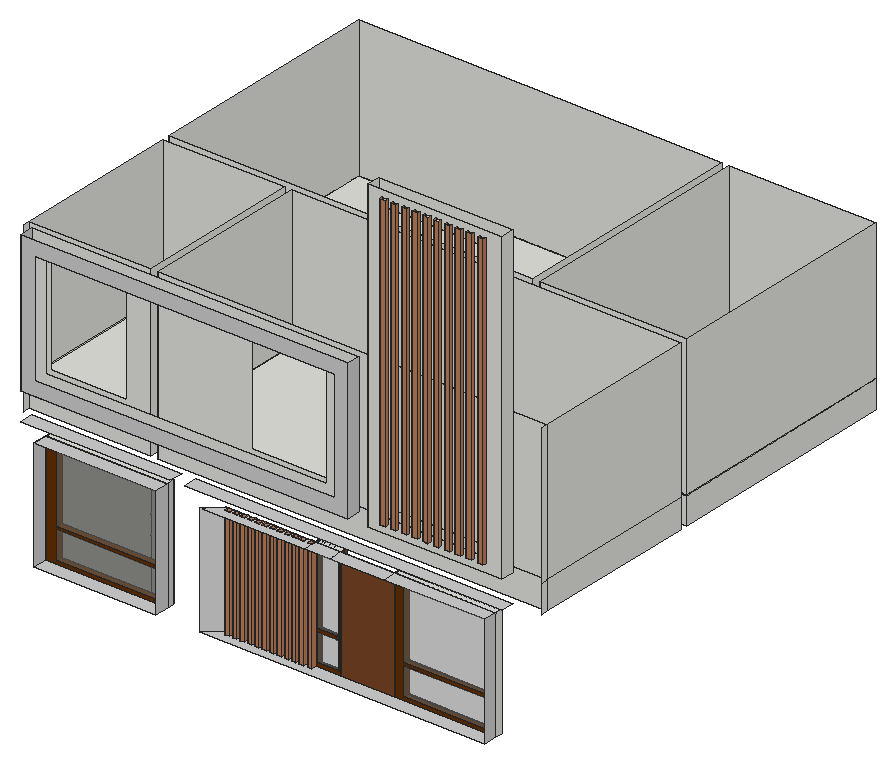
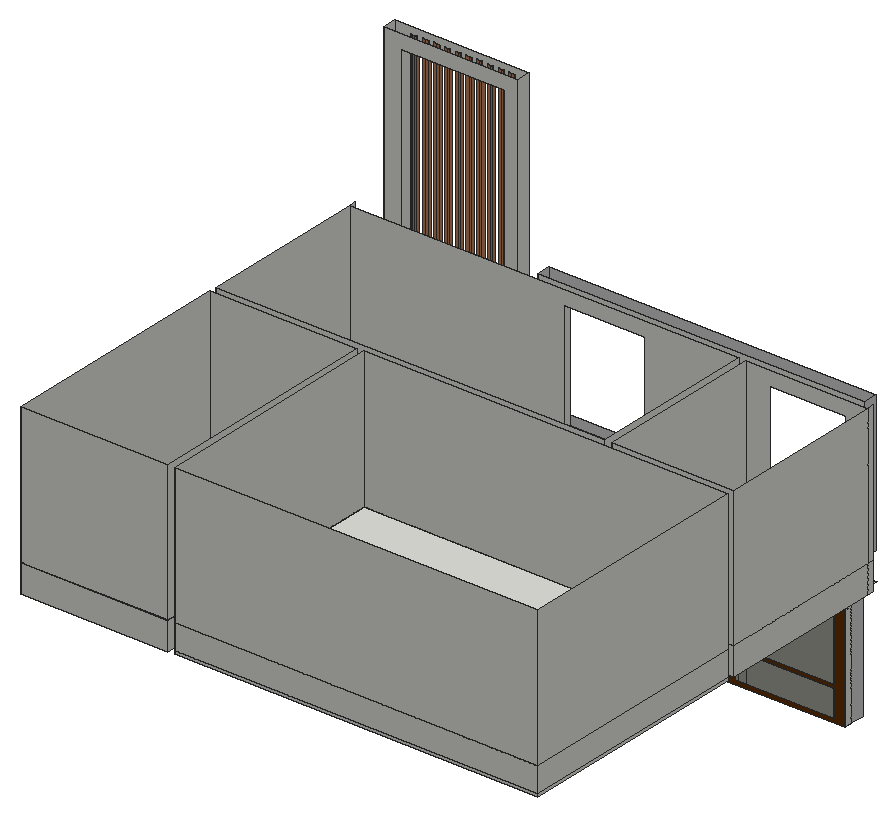
# SketchUp Ruby script. Lengths in inches.
U = 1.inch
M = Sketchup.active_model
def pt(a) = Geom::Point3d.new(a.map { |v| v * U })
def face(e, loops, mat)
  f = e.add_face(loops[0].map { |a| pt(a) })
  loops[1..].each { |l| e.add_face(l.map { |a| pt(a) }).erase! }
  f.material = f.back_material = mat if mat
  f
end
# faces: each face lists its corners as indices into pts; further lists are holes
def faces(e, pts, list, mat = nil) = list.each { |f| face(e, (f[0].is_a?(Array) ? f : [f]).map { |l| l.map { |i| pts[i] } }, mat) }
# xy, xz, yz: faces in a plane at the given z, y or x. An outline is a flat list of corners, or four numbers for a rectangle; further outlines are holes
def ring(l) = l.size == 4 ? [[l[0], l[1]], [l[2], l[1]], [l[2], l[3]], [l[0], l[3]]] : l.each_slice(2).to_a
def flat(e, list, mat, &to3) = list.each { |f| face(e, (f[0].is_a?(Array) ? f : [f]).map { |l| ring(l).map { |u, v| to3.(u, v) } }, mat) }
def xy(e, z, list, mat = nil) = flat(e, list, mat) { |x, y| [x, y, z] }
def xz(e, y, list, mat = nil) = flat(e, list, mat) { |x, z| [x, y, z] }
def yz(e, x, list, mat = nil) = flat(e, list, mat) { |y, z| [x, y, z] }
def lines(e, pts, list) = list.each { |a, b| e.add_line(pt(pts[a]), pt(pts[b])) }
# prism: a flat outline (further loops are holes) pulled along v
def prism(e, loops, v, mat = nil)
  f = face(e, loops, mat); d = Geom::Vector3d.new(v.map { |x| x * U })
  f.pushpull(f.normal.samedirection?(d) ? d.length : -d.length)
end
def box(e, o, s, mat = nil) = prism(e, [[o, [o[0] + s[0], o[1], o[2]], [o[0] + s[0], o[1] + s[1], o[2]], [o[0], o[1] + s[1], o[2]]]], [0, 0, s[2]], mat)
def at(x, y, z, deg = 0) = Geom::Transformation.translation(pt([x, y, z])) * Geom::Transformation.rotation(ORIGIN, Z_AXIS, deg.degrees)
def axes(o, x, y, z) = Geom::Transformation.new([*x, 0, *y, 0, *z, 0, *pt(o).to_a, 1])
def part(name) = M.definitions.add(name)
# library, detail: a bought-in or finely detailed component or shape, given as its bounding box
def library(name, o, s) = part(name).tap { |d| box(d.entities, o, s) }
def detail(e, o, s) = box(e.add_group.entities, o, s)
def put(e, d, t, mat = nil) = e.add_instance(d, t).tap { |i| i.material = mat if mat }
def group(e, t, mat = nil) = e.add_group.tap { |g| g.transformation = t; g.material = mat if mat }.entities
root = M.entities
M.materials.add("[Blinds Vertical Stripe Gray]").color = [160, 160, 152]
M.materials.add("[Carrera Marble]").color = [207, 207, 207]
M.materials.add("[Color A08]").color = [102, 48, 0]
M.materials.add("[Translucent Glass Gray]").color = [128, 128, 128]
M.materials["[Translucent Glass Gray]"].alpha = 0.5
M.materials.add("[Wood Veneer 01]").color = [120, 70, 37]
M.materials.add("[Wood Veneer 02]").color = [190, 128, 91]
c1 = part("Group\#3")
xy(c1.entities,0,[[0,0,42.75,0.0625],[0,0.0625,42.75,4.0625]],"[Color A08]")
xy(c1.entities,3.85,[[3.85,0,38.9,0.0625],[3.85,0.0625,38.9,4.0625]],"[Color A08]")
xy(c1.entities,34.99,[[3.85,0,38.9,0.0625],[3.85,0.0625,38.9,4.0625]],"[Color A08]")
xy(c1.entities,37.8125,[[3.85,0,38.9,0.0625],[3.85,0.0625,38.9,4.0625]],"[Color A08]")
xy(c1.entities,119.4,[[3.85,0,38.9,0.0625],[3.85,0.0625,38.9,4.0625]],"[Color A08]")
xy(c1.entities,123.25,[[0,0,42.75,0.0625],[0,0.0625,42.75,4.0625]],"[Color A08]")
xz(c1.entities,0,[[[0,0,42.75,123.25],[3.85,3.85,3.85,34.99,38.9,34.99,38.9,37.8125,3.85,37.8125,3.85,119.4,38.9,119.4,38.9,3.85]]],"[Color A08]")
xz(c1.entities,0.0625,[[[0,0,42.75,123.25],[3.85,3.85,3.85,34.99,38.9,34.99,38.9,37.8125,3.85,37.8125,3.85,119.4,38.9,119.4,38.9,3.85]]],"[Color A08]")
xz(c1.entities,0.0625,[[3.85,3.85,38.9,34.99],[3.85,37.8125,38.9,119.4]],"[Translucent Glass Gray]")
xz(c1.entities,4.0625,[[[0,0,42.75,123.25],[3.85,3.85,38.9,3.85,38.9,119.4,3.85,119.4,3.85,37.8125,38.9,37.8125,38.9,34.99,3.85,34.99]]],"[Color A08]")
yz(c1.entities,0,[[0,0,0.0625,123.25],[0.0625,0,4.0625,123.25]],"[Color A08]")
yz(c1.entities,3.85,[[0,3.85,0.0625,34.99],[0.0625,3.85,4.0625,34.99],[0,37.8125,0.0625,119.4],[0.0625,37.8125,4.0625,119.4]],"[Color A08]")
yz(c1.entities,38.9,[[0,3.85,0.0625,34.99],[0.0625,3.85,4.0625,34.99],[0,34.99,0.0625,37.8125],[0.0625,34.99,4.0625,37.8125],[0,37.8125,0.0625,119.4],
  [0.0625,37.8125,4.0625,119.4]],"[Color A08]")
yz(c1.entities,42.75,[[0,0,0.0625,123.25],[0.0625,0,4.0625,123.25]],"[Color A08]")
c2 = part("Group\#4")
xy(c2.entities,0,[[0,0,42.75,0.0625],[0,0.0625,42.75,4.0625]],"[Color A08]")
xy(c2.entities,3.85,[[3.85,0,38.9,0.0625],[3.85,0.0625,38.9,4.0625]],"[Color A08]")
xy(c2.entities,34.99,[[3.85,0,38.9,0.0625],[3.85,0.0625,38.9,4.0625]],"[Color A08]")
xy(c2.entities,37.8125,[[3.85,0,38.9,0.0625],[3.85,0.0625,38.9,4.0625]],"[Color A08]")
xy(c2.entities,119.4,[[3.85,0,38.9,0.0625],[3.85,0.0625,38.9,4.0625]],"[Color A08]")
xy(c2.entities,123.25,[[0,0,42.75,0.0625],[0,0.0625,42.75,4.0625]],"[Color A08]")
xz(c2.entities,0,[[[0,0,42.75,123.25],[3.85,3.85,3.85,34.99,38.9,34.99,38.9,37.8125,3.85,37.8125,3.85,119.4,38.9,119.4,38.9,3.85]]],"[Color A08]")
xz(c2.entities,0.0625,[[[0,0,42.75,123.25],[3.85,3.85,3.85,34.99,38.9,34.99,38.9,37.8125,3.85,37.8125,3.85,119.4,38.9,119.4,38.9,3.85]]],"[Color A08]")
xz(c2.entities,0.0625,[[3.85,3.85,38.9,34.99],[3.85,37.8125,38.9,119.4]],"[Translucent Glass Gray]")
xz(c2.entities,4.0625,[[[0,0,42.75,123.25],[3.85,3.85,38.9,3.85,38.9,119.4,3.85,119.4,3.85,37.8125,38.9,37.8125,38.9,34.99,3.85,34.99]]],"[Color A08]")
yz(c2.entities,0,[[0,0,0.0625,123.25],[0.0625,0,4.0625,123.25]],"[Color A08]")
yz(c2.entities,3.85,[[0,3.85,0.0625,34.99],[0.0625,3.85,4.0625,34.99],[0,37.8125,0.0625,119.4],[0.0625,37.8125,4.0625,119.4]],"[Color A08]")
yz(c2.entities,38.9,[[0,3.85,0.0625,34.99],[0.0625,3.85,4.0625,34.99],[0,34.99,0.0625,37.8125],[0.0625,34.99,4.0625,37.8125],[0,37.8125,0.0625,119.4],
  [0.0625,37.8125,4.0625,119.4]],"[Color A08]")
yz(c2.entities,42.75,[[0,0,0.0625,123.25],[0.0625,0,4.0625,123.25]],"[Color A08]")
xy(root,297,[[43.1875,102.75,148.25,108.75],[276.03,102.75,297.76,108.75],[344.2,102.75,431.1875,108.75]])
xy(root,297,[[43.1875,90.75,148.25,102.75],[185.91,90.75,431.1875,90.75,431.1875,102.75,276.03,102.75,276.03,98.5625,272.2,98.5625,272.2,102.75,268.97,102.75,268.97,98.5625,265.14,98.5625,265.14,102.75,262.54,102.75,262.54,98.5625,258.71,98.5625,258.71,102.75,256.16,102.75,256.16,98.5625,252.33,98.5625,252.33,102.75,249.79,102.75,249.79,98.5625,245.96,98.5625,245.96,102.75,243.41,102.75,243.41,98.5625,239.58,98.5625,239.58,102.75,237.04,102.75,237.04,98.5625,233.21,98.5625,233.21,102.75,230.66,102.75,230.66,98.5625,226.83,98.5625,226.83,102.75,224.29,102.75,224.29,98.5625,220.46,98.5625,220.46,102.75,217.91,102.75,217.91,98.5625,214.08,98.5625,214.08,102.75,211.54,102.75,211.54,98.5625,207.71,98.5625,207.71,102.75,205.16,102.75,205.16,98.5625,201.33,98.5625,201.33,102.75,198.8125,102.75]],"[Carrera Marble]")
xy(root,297,[[201.33,98.5625,205.16,102.75],[207.71,98.5625,211.54,102.75],[214.08,98.5625,217.91,102.75],[220.46,98.5625,224.29,102.75],[226.83,98.5625,230.66,102.75],
  [233.21,98.5625,237.04,102.75],[239.58,98.5625,243.41,102.75],[245.96,98.5625,249.79,102.75],[252.33,98.5625,256.16,102.75],[258.71,98.5625,262.54,102.75],
  [265.14,98.5625,268.97,102.75],[272.2,98.5625,276.03,102.75]],"[Wood Veneer 02]")
xy(root,393,[[43.1875,102.75,148.25,108.75],[276.03,102.75,297.76,108.75],[344.2,102.75,431.1875,108.75]])
xy(root,393,[[43.1875,90.75,148.25,102.75],[185.91,90.75,198.8125,102.75,201.33,102.75,201.33,98.5625,205.16,98.5625,205.16,102.75,207.71,102.75,207.71,98.5625,211.54,98.5625,211.54,102.75,214.08,102.75,214.08,98.5625,217.91,98.5625,217.91,102.75,220.46,102.75,220.46,98.5625,224.29,98.5625,224.29,102.75,226.83,102.75,226.83,98.5625,230.66,98.5625,230.66,102.75,233.21,102.75,233.21,98.5625,237.04,98.5625,237.04,102.75,239.58,102.75,239.58,98.5625,243.41,98.5625,243.41,102.75,245.96,102.75,245.96,98.5625,249.79,98.5625,249.79,102.75,252.33,102.75,252.33,98.5625,256.16,98.5625,256.16,102.75,258.71,102.75,258.71,98.5625,262.54,98.5625,262.54,102.75,265.14,102.75,265.14,98.5625,268.97,98.5625,268.97,102.75,272.2,102.75,272.2,98.5625,276.03,98.5625,276.03,90.75],[276.03,90.75,297.76,102.75],[297.76,90.75,344.2,102.75],[344.2,90.75,431.1875,102.75]],"[Carrera Marble]")
xy(root,393,[[201.33,98.5625,205.16,102.75],[207.71,98.5625,211.54,102.75],[214.08,98.5625,217.91,102.75],[220.46,98.5625,224.29,102.75],[226.83,98.5625,230.66,102.75],
  [233.21,98.5625,237.04,102.75],[239.58,98.5625,243.41,102.75],[245.96,98.5625,249.79,102.75],[252.33,98.5625,256.16,102.75],[258.71,98.5625,262.54,102.75],
  [265.14,98.5625,268.97,102.75],[272.2,98.5625,276.03,102.75]],"[Wood Veneer 02]")
xy(root,405,[[31.1875,90.75,160.25,102.75],[173,90.75,445.6875,102.75]],"[Carrera Marble]")
xy(root,407.25,[[24.5,258.8125,337.8125,463]])
xy(root,428.5625,[[343.8125,258.8125,470.5,463]])
xy(root,429,[[330,90.75,445.6875,102.75],[24.5,108.75,129.23,252.8125],[135.23,108.75,470.5,252.8125],[24.5,258.8125,337.8125,463],[343.8125,258.8125,470.5,463]])
xy(root,429,[[31.25,90.75,312.9375,102.75]],"[Carrera Marble]")
xy(root,436.0625,[[342.74,88.5,347.3,90.75],[351.99,88.5,356.55,90.75],[361.24,88.5,365.8,90.75],[370.49,88.5,375.05,90.75],[379.74,88.5,384.3,90.75],
  [388.99,88.5,393.55,90.75],[398.24,88.5,402.8,90.75],[407.49,88.5,412.05,90.75],[416.93,88.5,421.49,90.75],[427.11,88.5,431.68,90.75]],"[Wood Veneer 02]")
xz(root,88.5,[[342.74,436.0625,347.3,687.5],[351.99,436.0625,356.55,687.5],[361.24,436.0625,365.8,687.5],[370.49,436.0625,375.05,687.5],[379.74,436.0625,384.3,687.5],
  [388.99,436.0625,393.55,687.5],[398.24,436.0625,402.8,687.5],[407.49,436.0625,412.05,687.5],[416.93,436.0625,421.49,687.5],[427.11,436.0625,431.68,687.5]],"[Wood Veneer 02]")
xz(root,90.75,[[[330,429,445.6875,693],[342.74,436.0625,342.74,441,341.75,441,341.75,681,342.74,681,342.74,687.5,347.3,687.5,347.3,681,351.99,681,351.99,687.5,356.55,687.5,356.55,681,361.24,681,361.24,687.5,365.8,687.5,365.8,681,370.49,681,370.49,687.5,375.05,687.5,375.05,681,379.74,681,379.74,687.5,384.3,687.5,384.3,681,388.99,681,388.99,687.5,393.55,687.5,393.55,681,398.24,681,398.24,687.5,402.8,687.5,402.8,681,407.49,681,407.49,687.5,412.05,687.5,412.05,681,416.93,681,416.93,687.5,421.49,687.5,421.49,681,427.11,681,427.11,687.5,431.68,687.5,431.68,436.0625,427.11,436.0625,427.11,441,421.49,441,421.49,436.0625,416.93,436.0625,416.93,441,412.05,441,412.05,436.0625,407.49,436.0625,407.49,441,402.8,441,402.8,436.0625,398.24,436.0625,398.24,441,393.55,441,393.55,436.0625,388.99,436.0625,388.99,441,384.3,441,384.3,436.0625,379.74,436.0625,379.74,441,375.05,441,375.05,436.0625,370.49,436.0625,370.49,441,365.8,441,365.8,436.0625,361.24,436.0625,361.24,441,356.55,441,356.55,436.0625,351.99,436.0625,351.99,441,347.3,441,347.3,436.0625]]])
xz(root,90.75,[[[31.25,429,312.9375,549],[43.25,441,301.84,537]]],"[Carrera Marble]")
xz(root,90.75,[[342.74,436.0625,347.3,441],[351.99,436.0625,356.55,441],[361.24,436.0625,365.8,441],[370.49,436.0625,375.05,441],[379.74,436.0625,384.3,441],
  [388.99,436.0625,393.55,441],[398.24,436.0625,402.8,441],[407.49,436.0625,412.05,441],[416.93,436.0625,421.49,441],[427.11,436.0625,427.11,441,431.1875,441,431.1875,687.5,431.68,687.5,431.68,436.0625]],"[Wood Veneer 02]")
xz(root,98.5625,[[201.33,297,205.16,393],[207.71,297,211.54,393],[214.08,297,217.91,393],[220.46,297,224.29,393],[226.83,297,230.66,393],
  [233.21,297,237.04,393],[239.58,297,243.41,393],[245.96,297,249.79,393],[252.33,297,256.16,393],[258.71,297,262.54,393],
  [265.14,297,268.97,393],[272.2,297,276.03,393]],"[Wood Veneer 02]")
xz(root,102.75,[[[31.25,429,312.9375,549],[43.25,441,285.875,537]],[[330,429,445.6875,693],[341.75,441,431.1875,681]]])
xz(root,102.75,[[198.8125,297,201.33,393],[205.16,297,207.71,393],[211.54,297,214.08,393],[217.91,297,220.46,393],[224.29,297,226.83,393],
  [230.66,297,233.21,393],[237.04,297,239.58,393],[243.41,297,245.96,393],[249.79,297,252.33,393],[256.16,297,258.71,393],
  [262.54,297,265.14,393],[268.97,297,272.2,393],[297.76,297,344.2,393]],"[Wood Veneer 01]")
xz(root,102.75,[[201.33,297,205.16,393],[207.71,297,211.54,393],[214.08,297,217.91,393],[220.46,297,224.29,393],[226.83,297,230.66,393],
  [233.21,297,237.04,393],[239.58,297,243.41,393],[245.96,297,249.79,393],[252.33,297,256.16,393],[258.71,297,262.54,393],
  [265.14,297,268.97,393],[272.2,297,276.03,393]],"[Wood Veneer 02]")
xz(root,108.75,[[24.5,405,129.23,429],[135.23,405,470.5,429],[[24.5,429,129.23,549],[43.25,441,108.92,537]],[[135.23,429,470.5,549],[215.87,441,285.875,537]]])
xz(root,108.75,[[43.1875,297,129.23,393],[129.23,297,135.23,393],[135.23,297,148.25,393]],"[Blinds Vertical Stripe Gray]")
xz(root,252.8125,[[24.5,405,129.23,429],[135.23,405,470.5,429],[24.5,429,129.23,549],[135.23,429,470.5,549]])
xz(root,258.8125,[[24.5,405,337.8125,407.25],[343.8125,405,470.5,428.5625],[24.5,407.25,94.98,429],[94.98,407.25,106.11,429],[106.11,407.25,337.8125,429],
  [343.8125,428.5625,429.375,429],[429.375,428.5625,432.3125,429],[432.3125,428.5625,470.5,429],[24.5,429,337.8125,549],[343.8125,429,470.5,549]])
xz(root,463,[[24.5,405,337.8125,407.25],[343.8125,405,470.5,428.5625],[24.5,407.25,337.8125,429],[343.8125,428.5625,470.5,429],[24.5,429,337.8125,549],
  [343.8125,429,470.5,549]])
yz(root,24.5,[[102.75,405,108.75,429],[108.75,405,252.8125,429],[258.8125,405,463,407.25],[258.8125,407.25,463,429],[102.75,429,108.75,549],
  [108.75,429,252.8125,549],[258.8125,429,463,549]])
yz(root,31.25,[[90.75,429,102.75,549]],"[Carrera Marble]")
yz(root,43.1875,[[102.75,297,108.75,393]])
yz(root,43.1875,[[90.75,297,102.75,393]],"[Carrera Marble]")
yz(root,129.23,[[108.75,405,252.8125,429],[108.75,429,252.8125,549]])
yz(root,135.23,[[108.75,405,252.8125,429],[108.75,429,252.8125,549]])
yz(root,148.25,[[90.75,297,102.75,393],[102.75,297,108.75,393]],"[Carrera Marble]")
yz(root,201.33,[[98.5625,297,102.75,393]],"[Wood Veneer 02]")
yz(root,205.16,[[98.5625,297,102.75,393]],"[Wood Veneer 02]")
yz(root,207.71,[[98.5625,297,102.75,393]],"[Wood Veneer 02]")
yz(root,211.54,[[98.5625,297,102.75,393]],"[Wood Veneer 02]")
yz(root,214.08,[[98.5625,297,102.75,393]],"[Wood Veneer 02]")
yz(root,217.91,[[98.5625,297,102.75,393]],"[Wood Veneer 02]")
yz(root,220.46,[[98.5625,297,102.75,393]],"[Wood Veneer 02]")
yz(root,224.29,[[98.5625,297,102.75,393]],"[Wood Veneer 02]")
yz(root,226.83,[[98.5625,297,102.75,393]],"[Wood Veneer 02]")
yz(root,230.66,[[98.5625,297,102.75,393]],"[Wood Veneer 02]")
yz(root,233.21,[[98.5625,297,102.75,393]],"[Wood Veneer 02]")
yz(root,237.04,[[98.5625,297,102.75,393]],"[Wood Veneer 02]")
yz(root,239.58,[[98.5625,297,102.75,393]],"[Wood Veneer 02]")
yz(root,243.41,[[98.5625,297,102.75,393]],"[Wood Veneer 02]")
yz(root,245.96,[[98.5625,297,102.75,393]],"[Wood Veneer 02]")
yz(root,249.79,[[98.5625,297,102.75,393]],"[Wood Veneer 02]")
yz(root,252.33,[[98.5625,297,102.75,393]],"[Wood Veneer 02]")
yz(root,256.16,[[98.5625,297,102.75,393]],"[Wood Veneer 02]")
yz(root,258.71,[[98.5625,297,102.75,393]],"[Wood Veneer 02]")
yz(root,262.54,[[98.5625,297,102.75,393]],"[Wood Veneer 02]")
yz(root,265.14,[[98.5625,297,102.75,393]],"[Wood Veneer 02]")
yz(root,268.97,[[98.5625,297,102.75,393]],"[Wood Veneer 02]")
yz(root,272.2,[[98.5625,297,102.75,393]],"[Wood Veneer 02]")
yz(root,276.03,[[102.75,297,108.75,393]],"[Wood Veneer 01]")
yz(root,276.03,[[98.5625,297,102.75,393]],"[Wood Veneer 02]")
yz(root,297.76,[[102.75,297,108.75,393]],"[Wood Veneer 01]")
yz(root,312.9375,[[90.75,429,102.75,549]],"[Carrera Marble]")
yz(root,330,[[90.75,429,102.75,693]])
yz(root,337.8125,[[258.8125,405,463,407.25],[258.8125,407.25,463,429],[258.8125,429,463,549]])
yz(root,342.74,[[88.5,436.0625,90.75,687.5]],"[Wood Veneer 02]")
yz(root,343.8125,[[258.8125,405,463,428.5625],[258.8125,428.5625,463,429],[258.8125,429,463,549]])
yz(root,344.2,[[102.75,297,108.75,393]],"[Wood Veneer 01]")
yz(root,347.3,[[88.5,436.0625,90.75,687.5]],"[Wood Veneer 02]")
yz(root,351.99,[[88.5,436.0625,90.75,687.5]],"[Wood Veneer 02]")
yz(root,356.55,[[88.5,436.0625,90.75,687.5]],"[Wood Veneer 02]")
yz(root,361.24,[[88.5,436.0625,90.75,687.5]],"[Wood Veneer 02]")
yz(root,365.8,[[88.5,436.0625,90.75,687.5]],"[Wood Veneer 02]")
yz(root,370.49,[[88.5,436.0625,90.75,687.5]],"[Wood Veneer 02]")
yz(root,375.05,[[88.5,436.0625,90.75,687.5]],"[Wood Veneer 02]")
yz(root,379.74,[[88.5,436.0625,90.75,687.5]],"[Wood Veneer 02]")
yz(root,384.3,[[88.5,436.0625,90.75,687.5]],"[Wood Veneer 02]")
yz(root,388.99,[[88.5,436.0625,90.75,687.5]],"[Wood Veneer 02]")
yz(root,393.55,[[88.5,436.0625,90.75,687.5]],"[Wood Veneer 02]")
yz(root,398.24,[[88.5,436.0625,90.75,687.5]],"[Wood Veneer 02]")
yz(root,402.8,[[88.5,436.0625,90.75,687.5]],"[Wood Veneer 02]")
yz(root,407.49,[[88.5,436.0625,90.75,687.5]],"[Wood Veneer 02]")
yz(root,412.05,[[88.5,436.0625,90.75,687.5]],"[Wood Veneer 02]")
yz(root,416.93,[[88.5,436.0625,90.75,687.5]],"[Wood Veneer 02]")
yz(root,421.49,[[88.5,436.0625,90.75,687.5]],"[Wood Veneer 02]")
yz(root,427.11,[[88.5,436.0625,90.75,687.5]],"[Wood Veneer 02]")
yz(root,431.1875,[[102.75,297,108.75,393]])
yz(root,431.1875,[[90.75,297,102.75,393]],"[Carrera Marble]")
yz(root,431.68,[[88.5,436.0625,90.75,687.5]],"[Wood Veneer 02]")
yz(root,445.6875,[[90.75,429,102.75,693]])
yz(root,470.5,[[102.75,405,108.75,429],[108.75,405,252.8125,429],[258.8125,405,463,428.5625],[258.8125,428.5625,463,429],[102.75,429,108.75,549],
  [108.75,429,252.8125,549],[258.8125,429,463,549]])
p = [[185.91,90.75,297],[198.8125,102.75,297],[198.8125,102.75,393],[185.91,90.75,393]]
faces(root,p,[[0,1,2,3]],"[Carrera Marble]")
put(root,c1,axes([344.2,102.75,297],[2.03468,0,0],[0,1.14716,0],[0,0,0.7789]))
put(root,c2,axes([275.71,102.75,297],[0.51591,0,0],[0,0.7,0],[0,0,0.777]))
put(root,c1,axes([43.1875,102.75,297],[2.4576,0,0],[0,1.687,0],[0,0,0.777]))
